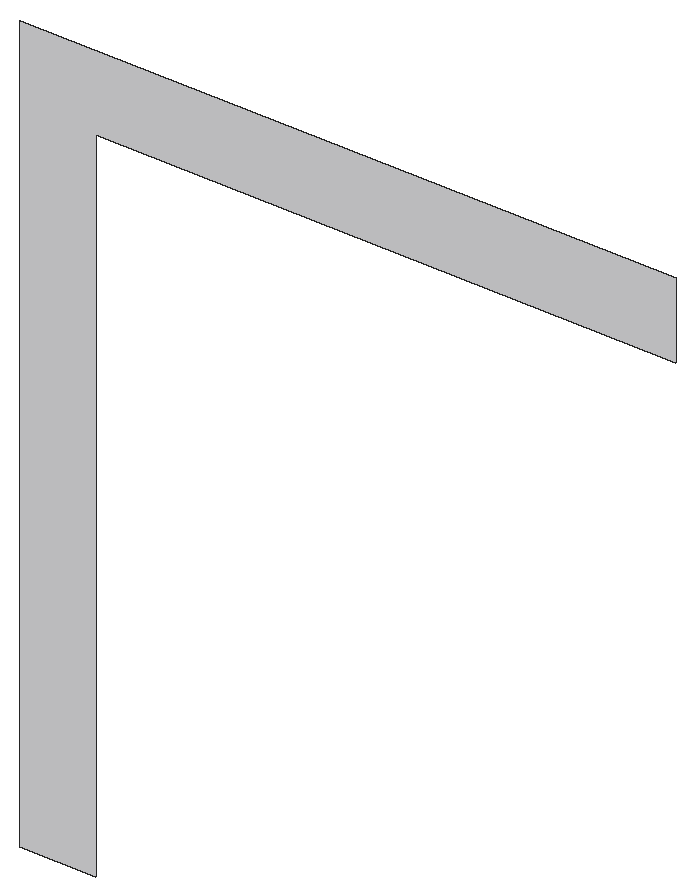
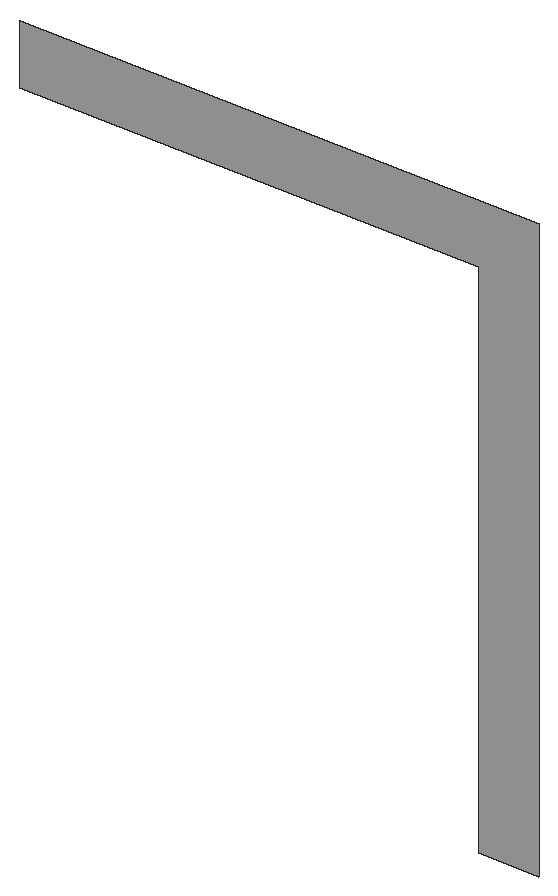
# SketchUp Ruby script. Lengths in inches.
U = 1.inch
M = Sketchup.active_model
def pt(a) = Geom::Point3d.new(a.map { |v| v * U })
def face(e, loops, mat)
  f = e.add_face(loops[0].map { |a| pt(a) })
  loops[1..].each { |l| e.add_face(l.map { |a| pt(a) }).erase! }
  f.material = f.back_material = mat if mat
  f
end
# faces: each face lists its corners as indices into pts; further lists are holes
def faces(e, pts, list, mat = nil) = list.each { |f| face(e, (f[0].is_a?(Array) ? f : [f]).map { |l| l.map { |i| pts[i] } }, mat) }
# xy, xz, yz: faces in a plane at the given z, y or x. An outline is a flat list of corners, or four numbers for a rectangle; further outlines are holes
def ring(l) = l.size == 4 ? [[l[0], l[1]], [l[2], l[1]], [l[2], l[3]], [l[0], l[3]]] : l.each_slice(2).to_a
def flat(e, list, mat, &to3) = list.each { |f| face(e, (f[0].is_a?(Array) ? f : [f]).map { |l| ring(l).map { |u, v| to3.(u, v) } }, mat) }
def xy(e, z, list, mat = nil) = flat(e, list, mat) { |x, y| [x, y, z] }
def xz(e, y, list, mat = nil) = flat(e, list, mat) { |x, z| [x, y, z] }
def yz(e, x, list, mat = nil) = flat(e, list, mat) { |y, z| [x, y, z] }
def lines(e, pts, list) = list.each { |a, b| e.add_line(pt(pts[a]), pt(pts[b])) }
# prism: a flat outline (further loops are holes) pulled along v
def prism(e, loops, v, mat = nil)
  f = face(e, loops, mat); d = Geom::Vector3d.new(v.map { |x| x * U })
  f.pushpull(f.normal.samedirection?(d) ? d.length : -d.length)
end
def box(e, o, s, mat = nil) = prism(e, [[o, [o[0] + s[0], o[1], o[2]], [o[0] + s[0], o[1] + s[1], o[2]], [o[0], o[1] + s[1], o[2]]]], [0, 0, s[2]], mat)
def at(x, y, z, deg = 0) = Geom::Transformation.translation(pt([x, y, z])) * Geom::Transformation.rotation(ORIGIN, Z_AXIS, deg.degrees)
def axes(o, x, y, z) = Geom::Transformation.new([*x, 0, *y, 0, *z, 0, *pt(o).to_a, 1])
def part(name) = M.definitions.add(name)
# library, detail: a bought-in or finely detailed component or shape, given as its bounding box
def library(name, o, s) = part(name).tap { |d| box(d.entities, o, s) }
def detail(e, o, s) = box(e.add_group.entities, o, s)
def put(e, d, t, mat = nil) = e.add_instance(d, t).tap { |i| i.material = mat if mat }
def group(e, t, mat = nil) = e.add_group.tap { |g| g.transformation = t; g.material = mat if mat }.entities
root = M.entities
M.materials.add("[Blinds Vertical Pattern]").color = [232, 232, 234]
xz(root,225.17,[[176.75,137.875,189.02,137.875,189.02,245.5,283.04,245.5,283.04,257.875,176.75,257.875]],"[Blinds Vertical Pattern]")
